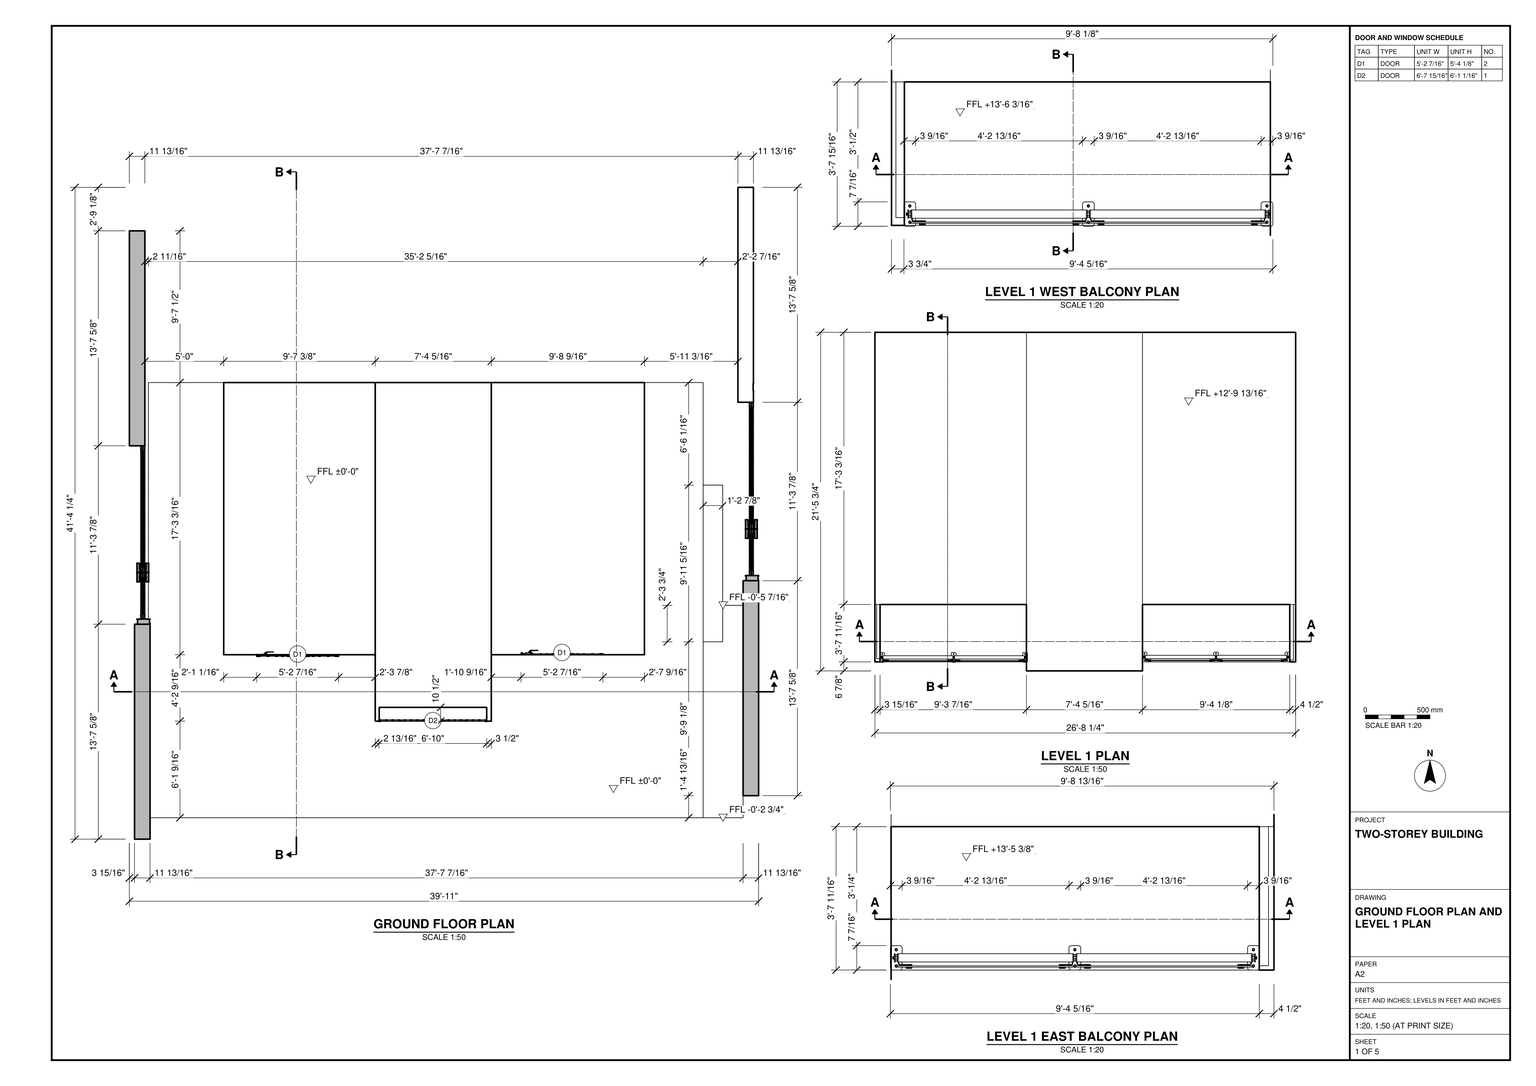
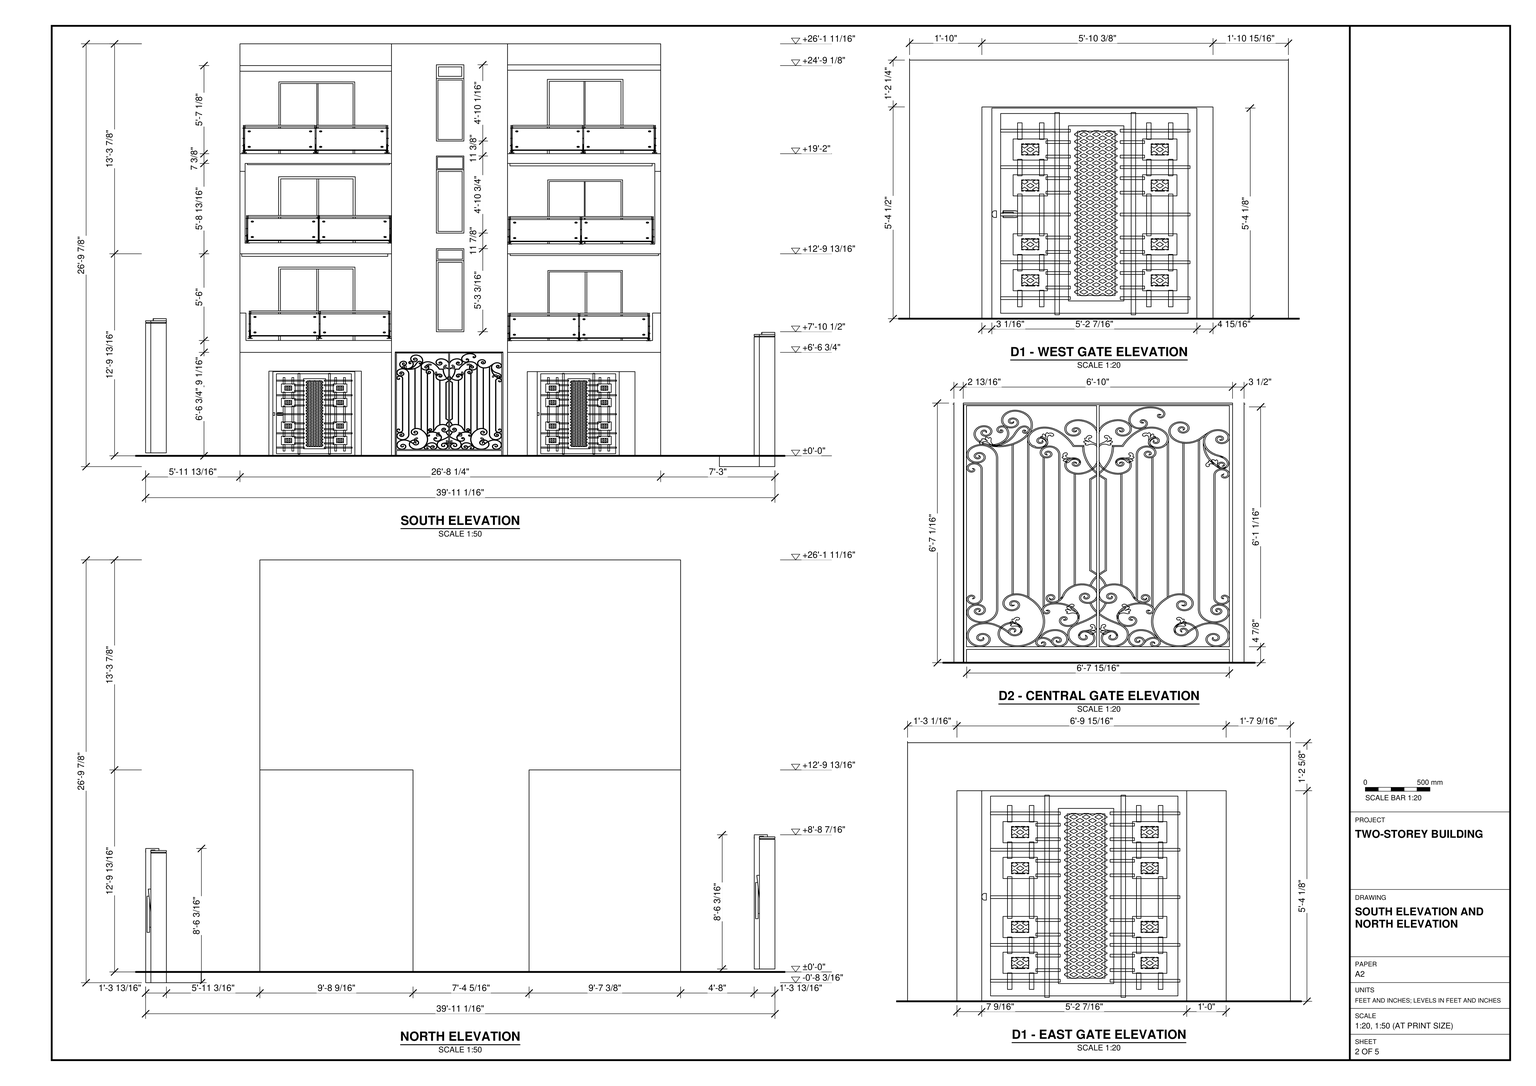
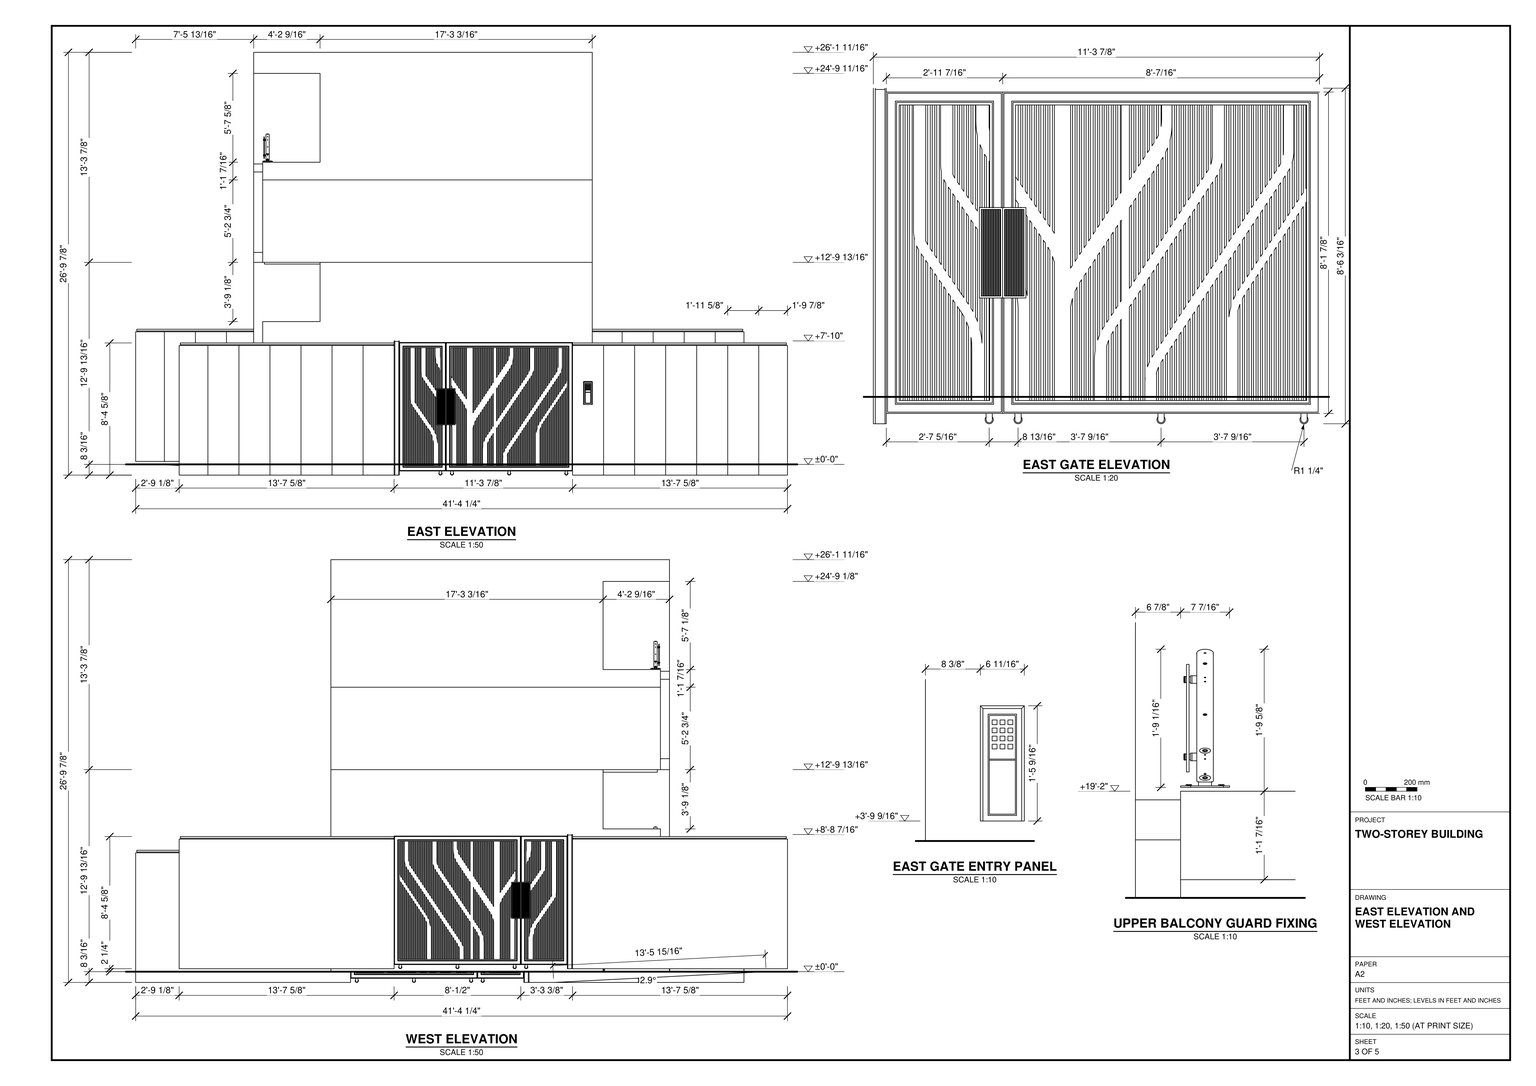
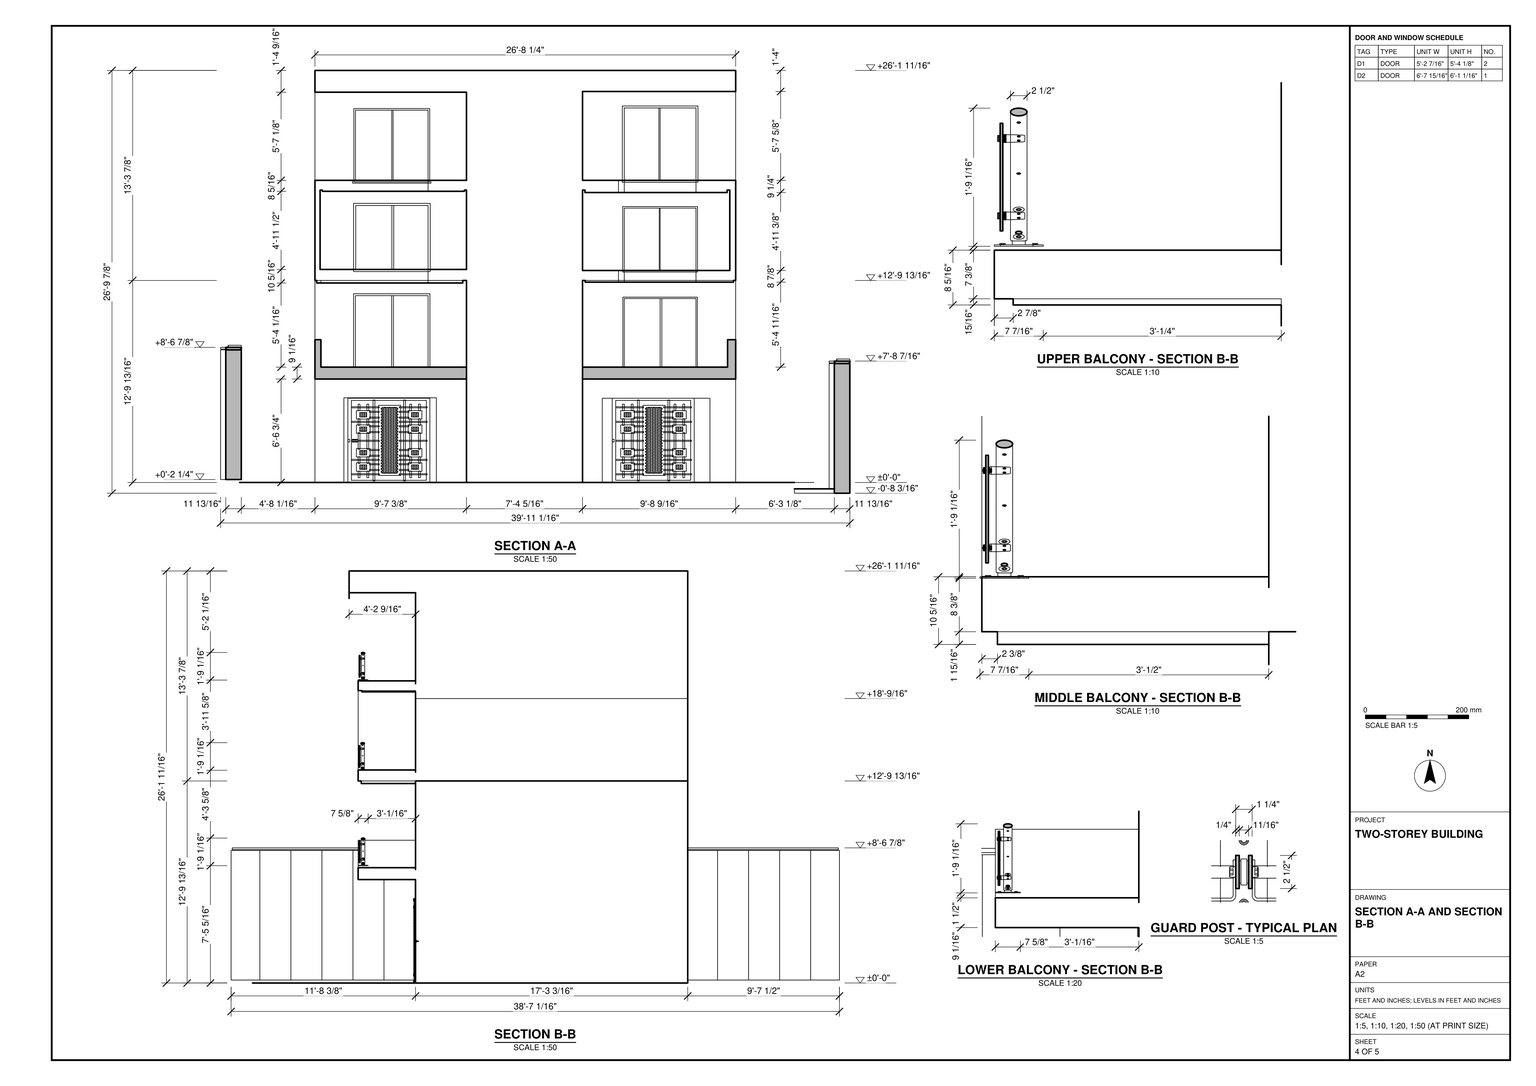
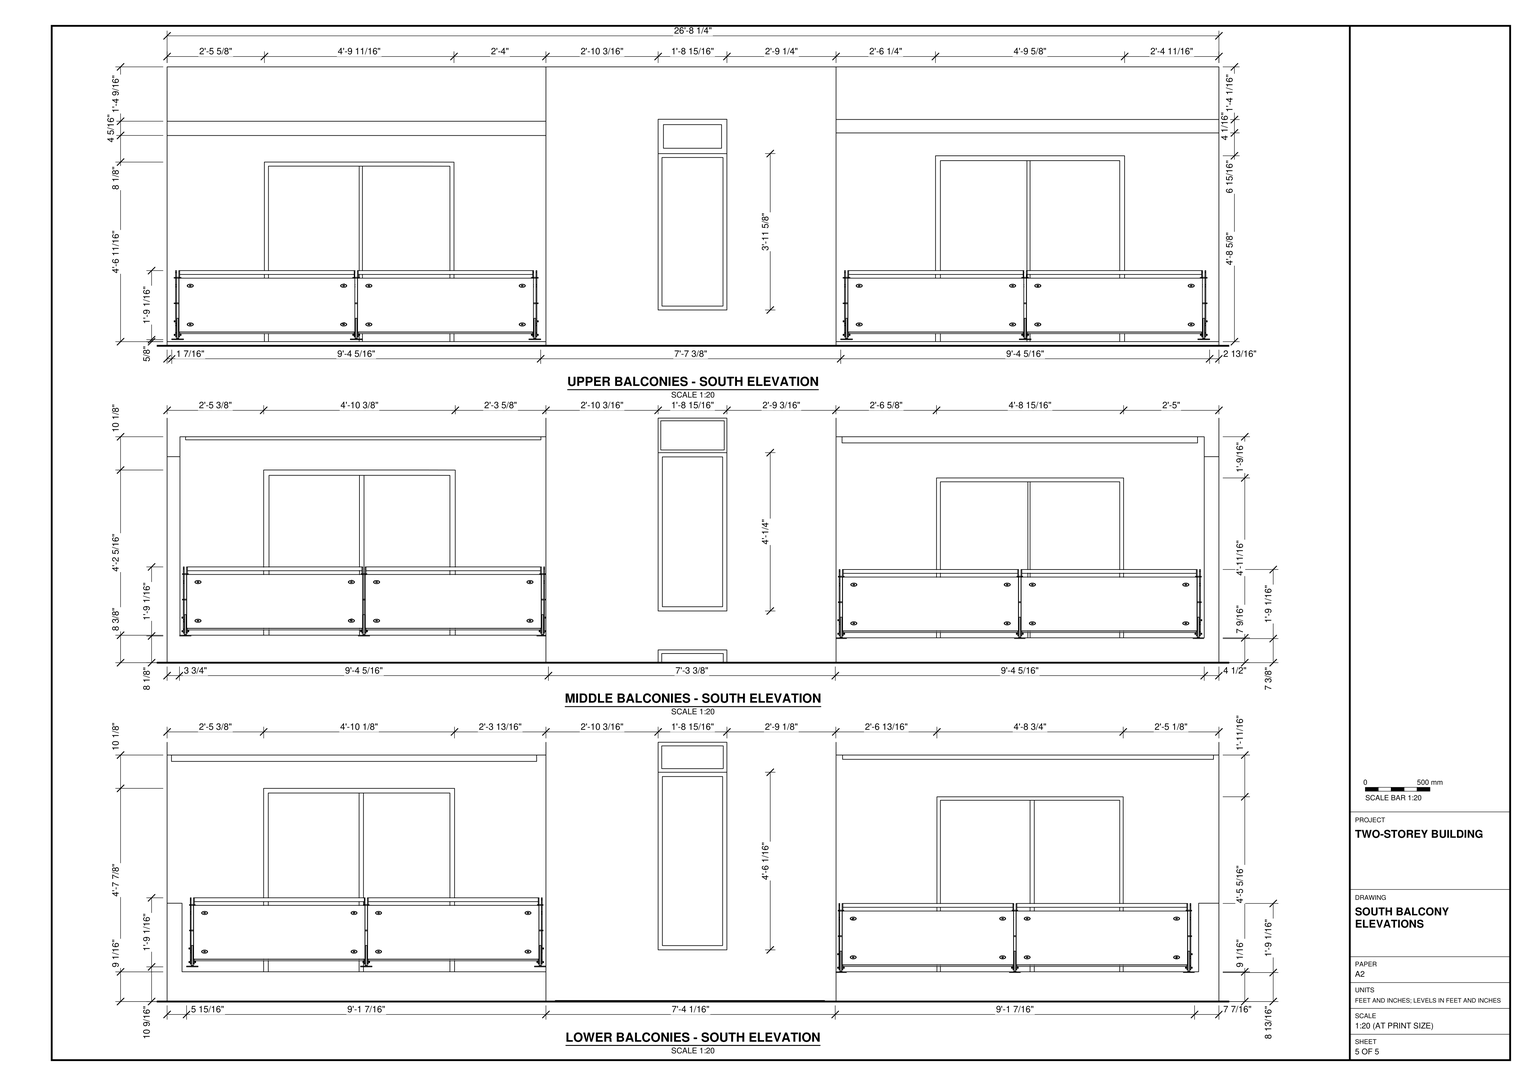
Build the two-storey building and its gated site in SketchUp using task_files/diagram_01.pdf. Work in feet and inches. Set out the complete model, including the side boundary walls, to an overall width of 39'-11 1/16", depth of 41'-4 1/4" and height of 26'-9 7/8". Use ±0'-0" for the ground floor and +12'-9 13/16" for Level 1.

Follow the plans for the building footprint, the projection of the central entrance bay and the clearances between the building and the boundary walls. Model the walls, floor and balcony slabs, openings and flat roof with their thicknesses as drawn. On the south face, place the wider central gate between the two matching entrance gates. Follow the south elevation for the three balcony tiers on either side of the central bay, including the glazed openings behind the guards and the narrow windows in the central bay. Use the balcony details for the glass panels, posts and fixings.

Model the east and west boundary walls with their gate openings in the positions shown in plan. Follow the side elevations for the unequal gate leaves, branching bar pattern and east entry panel. Keep shell elements, gates and any furniture or joinery pieces in separate groups or components, and use components for repeated parts. Decor and loose items, if shown, may be any suitable library components. Save one SketchUp model as output_files/two_storey_building_with_balconies_and_gated_side_walls.skp.

# SketchUp Ruby script. Lengths in inches.
U = 1.inch
M = Sketchup.active_model
def pt(a) = Geom::Point3d.new(a.map { |v| v * U })
def face(e, loops, mat)
  f = e.add_face(loops[0].map { |a| pt(a) })
  loops[1..].each { |l| e.add_face(l.map { |a| pt(a) }).erase! }
  f.material = f.back_material = mat if mat
  f
end
# faces: each face lists its corners as indices into pts; further lists are holes
def faces(e, pts, list, mat = nil) = list.each { |f| face(e, (f[0].is_a?(Array) ? f : [f]).map { |l| l.map { |i| pts[i] } }, mat) }
# xy, xz, yz: faces in a plane at the given z, y or x. An outline is a flat list of corners, or four numbers for a rectangle; further outlines are holes
def ring(l) = l.size == 4 ? [[l[0], l[1]], [l[2], l[1]], [l[2], l[3]], [l[0], l[3]]] : l.each_slice(2).to_a
def flat(e, list, mat, &to3) = list.each { |f| face(e, (f[0].is_a?(Array) ? f : [f]).map { |l| ring(l).map { |u, v| to3.(u, v) } }, mat) }
def xy(e, z, list, mat = nil) = flat(e, list, mat) { |x, y| [x, y, z] }
def xz(e, y, list, mat = nil) = flat(e, list, mat) { |x, z| [x, y, z] }
def yz(e, x, list, mat = nil) = flat(e, list, mat) { |y, z| [x, y, z] }
def lines(e, pts, list) = list.each { |a, b| e.add_line(pt(pts[a]), pt(pts[b])) }
# prism: a flat outline (further loops are holes) pulled along v
def prism(e, loops, v, mat = nil)
  f = face(e, loops, mat); d = Geom::Vector3d.new(v.map { |x| x * U })
  f.pushpull(f.normal.samedirection?(d) ? d.length : -d.length)
end
def box(e, o, s, mat = nil) = prism(e, [[o, [o[0] + s[0], o[1], o[2]], [o[0] + s[0], o[1] + s[1], o[2]], [o[0], o[1] + s[1], o[2]]]], [0, 0, s[2]], mat)
def at(x, y, z, deg = 0) = Geom::Transformation.translation(pt([x, y, z])) * Geom::Transformation.rotation(ORIGIN, Z_AXIS, deg.degrees)
def axes(o, x, y, z) = Geom::Transformation.new([*x, 0, *y, 0, *z, 0, *pt(o).to_a, 1])
def part(name) = M.definitions.add(name)
# library, detail: a bought-in or finely detailed component or shape, given as its bounding box
def library(name, o, s) = part(name).tap { |d| box(d.entities, o, s) }
def detail(e, o, s) = box(e.add_group.entities, o, s)
def put(e, d, t, mat = nil) = e.add_instance(d, t).tap { |i| i.material = mat if mat }
def group(e, t, mat = nil) = e.add_group.tap { |g| g.transformation = t; g.material = mat if mat }.entities
root = M.entities
M.materials.add("0-370-55720370副本4").color = [155, 133, 94]
M.materials.add("1").color = [35, 24, 16]
M.materials.add("Niraj_Hair_Dark").color = [109, 109, 109]
M.materials.add("[0009_Linen]").color = [250, 240, 230]
M.materials.add("[0028_AntiqueWhite]").color = [250, 235, 215]
M.materials.add("[Asphalt New]").color = [67, 60, 62]
M.materials.add("[Metal Corrugated Shiny]16").color = [144, 125, 78]
M.materials.add("[Translucent Glass Gray]").color = [128, 128, 128]
M.materials["[Translucent Glass Gray]"].alpha = 0.5
M.materials.add("主石材1").color = [201, 201, 201]
c1 = library("2.Gate",[0,0,0],[31.23,2.83,52.14])
c2 = library("Driveway gate",[0.2,-91.45,-1.97],[10.04,135.85,102.19])
c3 = part("组\#15")
xy(c3.entities,-0.2,[[111.54,0,274.3125,11.88]],"0-370-55720370副本4")
xy(c3.entities,0.98,[[[111.54,0,274.3125,11.88],[112.13,0.59,273.72,11.29]]],"0-370-55720370副本4")
xy(c3.entities,1.57,[[112.13,0.59,273.72,11.29]],"0-370-55720370副本4")
xz(c3.entities,0,[[111.54,-0.2,274.3125,0.98]],"0-370-55720370副本4")
xz(c3.entities,0.59,[[112.13,0.98,273.72,1.57]],"0-370-55720370副本4")
xz(c3.entities,11.29,[[112.13,0.98,273.72,1.57]],"0-370-55720370副本4")
xz(c3.entities,11.88,[[111.54,-0.2,274.3125,0.98]],"0-370-55720370副本4")
yz(c3.entities,111.54,[[0,-0.2,11.88,0.98]],"0-370-55720370副本4")
yz(c3.entities,112.13,[[0.59,0.98,11.29,1.57]],"0-370-55720370副本4")
yz(c3.entities,273.72,[[0.59,0.98,11.29,1.57]],"0-370-55720370副本4")
yz(c3.entities,274.3125,[[0,-0.2,11.88,0.98]],"0-370-55720370副本4")
c4 = part("组\#14")
xy(c4.entities,15.75,[[0.39,-1.18,6.3,0.79]],"[Metal Corrugated Shiny]16")
xy(c4.entities,16.14,[[0,-1.18,6.69,0.79]],"[Metal Corrugated Shiny]16")
xz(c4.entities,-1.18,[[0,0,0.39,0,0.39,15.75,6.3,15.75,6.3,0,6.69,0,6.69,16.14,0,16.14]],"[Metal Corrugated Shiny]16")
xz(c4.entities,0.79,[[0.39,15.75,0,16.14,6.69,16.14,6.3,15.75]],"[Metal Corrugated Shiny]16")
yz(c4.entities,0,[[-1.18,0,-1.18,16.14,0.79,16.14,-0.2,8.07]],"[Metal Corrugated Shiny]16")
yz(c4.entities,0.39,[[-1.18,0,-0.2,7.875,0.79,15.75,-1.18,15.75]],"[Metal Corrugated Shiny]16")
yz(c4.entities,6.3,[[-1.18,0,-1.18,15.75,0.79,15.75,-0.2,7.875]],"[Metal Corrugated Shiny]16")
yz(c4.entities,6.69,[[-1.18,0,-0.2,8.07,0.79,16.14,-1.18,16.14]],"[Metal Corrugated Shiny]16")
p = [[0.39,-0.2,7.875],[0,-0.2,8.07],[0,-1.18,0],[0.39,-1.18,0],[6.69,-0.2,8.07],[6.3,-0.2,7.875],
  [6.69,-1.18,0],[6.3,-1.18,0],[0.39,0.79,15.75],[6.3,0.79,15.75],[0,0.79,16.14],[6.69,0.79,16.14]]
faces(c4.entities,p,[[0,1,2],[0,2,3],[4,5,6],[6,5,7],[8,1,0],[4,9,5],[8,10,1],[11,9,4]],"[Metal Corrugated Shiny]16")
c5 = part("组\#1730")
xy(c5.entities,19.61,[[-11.8125,0,151.8125,11.8125]],"主石材1")
xy(c5.entities,84.78,[[137.15,9.84,143.05,11.8125]],"[Metal Corrugated Shiny]16")
xy(c5.entities,110.36,[[-11.8125,0,151.8125,11.8125]],"主石材1")
xz(c5.entities,0,[[-11.8125,19.61,151.8125,110.36]],"主石材1")
xz(c5.entities,11.8125,[[[-11.8125,19.61,151.8125,110.36],[136.75,69.03,143.45,85.18]],[136.75,69.03,136.75,85.18,143.45,85.18,143.45,69.03,143.05,69.03,143.05,84.78,137.15,84.78,137.15,69.03]],"主石材1")
yz(c5.entities,-11.8125,[[0,19.61,11.8125,110.36]],"主石材1")
yz(c5.entities,137.15,[[11.8125,69.03,11.8125,84.78,9.84,84.78]],"[Metal Corrugated Shiny]16")
yz(c5.entities,143.05,[[11.8125,69.03,9.84,84.78,11.8125,84.78]],"[Metal Corrugated Shiny]16")
yz(c5.entities,151.8125,[[0,19.61,11.8125,110.36]],"主石材1")
p = [[137.15,9.84,84.78],[143.05,9.84,84.78],[143.05,11.8125,69.03],[137.15,11.8125,69.03],[142.26,9.94,84],[137.93,9.94,84],
  [137.93,11.71,69.82],[142.26,11.71,69.82],[142.08,10.73,77.71],[138.12,10.73,77.71],[138.12,10.75,77.55],[138.12,11.69,70],
  [142.08,11.69,70],[142.08,10.75,77.55],[142.08,9.96,83.82],[138.12,9.96,83.82],[139.71,10.04,83.1875],[139.71,10.125,82.53],
  [140.45,10.125,82.53],[140.45,10.04,83.1875],[138.51,10.18,82.05],[138.51,10.27,81.4],[139.25,10.27,81.4],[139.25,10.18,82.05],
  [139.71,10.33,80.92],[139.71,10.41,80.26],[140.45,10.41,80.26],[140.45,10.33,80.92],[138.51,10.47,79.79],[138.51,10.55,79.13],
  [139.25,10.55,79.13],[139.25,10.47,79.79],[138.51,10.04,83.1875],[138.51,10.125,82.53],[139.25,10.125,82.53],[139.25,10.04,83.1875],
  [140.91,10.18,82.05],[140.91,10.27,81.4],[141.65,10.27,81.4],[141.65,10.18,82.05],[138.51,10.33,80.92],[138.51,10.41,80.26],
  [139.25,10.41,80.26],[139.25,10.33,80.92],[140.91,10.33,80.92],[140.91,10.41,80.26],[141.65,10.41,80.26],[141.65,10.33,80.92],
  [140.91,10.47,79.79],[140.91,10.55,79.13],[141.65,10.55,79.13],[141.65,10.47,79.79],[140.91,10.04,83.1875],[140.91,10.125,82.53],
  [141.65,10.125,82.53],[141.65,10.04,83.1875],[139.71,10.18,82.05],[139.71,10.27,81.4],[140.45,10.27,81.4],[140.45,10.18,82.05],
  [139.71,10.47,79.79],[139.71,10.55,79.13],[140.45,10.55,79.13],[140.45,10.47,79.79]]
faces(c5.entities,p,[[[0,1,2,3],[4,5,6,7]],[[5,4,7,6],[8,9,10,11,12,13]],[10,13,12,11],[13,10,9,8],[[14,8,9,15],[16,17,18,19],[20,21,22,23],[24,25,26,27],[28,29,30,31],[32,33,34,35],[36,37,38,39],[40,41,42,43],[44,45,46,47],[48,49,50,51],[52,53,54,55],[56,57,58,59],[60,61,62,63]],[29,28,31,30],[61,60,63,62],[49,48,51,50],
  [41,40,43,42],[25,24,27,26],[45,44,47,46],[21,20,23,22],[57,56,59,58],[37,36,39,38],[33,32,35,34],[17,16,19,18],
  [53,52,55,54]],"[Metal Corrugated Shiny]16")
put(c5.entities,c4,at(136.75,12.99,69.03))
c6 = part("组\#263")
p = [[151.8125,11.8125,19.61],[151.8125,11.8125,110.36],[128.1875,11.8125,19.61],[128.1875,11.8125,110.36],[104.57,11.8125,19.61],[104.57,11.8125,110.36],
  [80.94,11.8125,19.61],[80.94,11.8125,110.36],[57.32,11.8125,19.61],[57.32,11.8125,110.36],[33.7,11.8125,19.61],[33.7,11.8125,110.36],
  [10.08,11.8125,19.61],[10.08,11.8125,110.36]]
lines(c6.entities,p,[[0,1],[0,2],[2,3],[4,5],[6,7],[8,9],[10,11],[12,13],[10,12],[8,10],[6,8],[4,6],
  [2,4]])
put(c6.entities,c3,axes([263.35,0,111.9375],[-1,0,0],[0,1,0],[0,0,-1]))
put(c6.entities,c5,at(0,0,0))
c7 = part("组\#1715")
xy(c7.entities,-0.2,[[111.54,0,274.3125,11.88]],"0-370-55720370副本4")
xy(c7.entities,0.98,[[[111.54,0,274.3125,11.88],[112.13,0.59,273.72,11.29]]],"0-370-55720370副本4")
xy(c7.entities,1.57,[[112.13,0.59,273.72,11.29]],"0-370-55720370副本4")
xz(c7.entities,0,[[111.54,-0.2,274.3125,0.98]],"0-370-55720370副本4")
xz(c7.entities,0.59,[[112.13,0.98,273.72,1.57]],"0-370-55720370副本4")
xz(c7.entities,11.29,[[112.13,0.98,273.72,1.57]],"0-370-55720370副本4")
xz(c7.entities,11.88,[[111.54,-0.2,274.3125,0.98]],"0-370-55720370副本4")
yz(c7.entities,111.54,[[0,-0.2,11.88,0.98]],"0-370-55720370副本4")
yz(c7.entities,112.13,[[0.59,0.98,11.29,1.57]],"0-370-55720370副本4")
yz(c7.entities,273.72,[[0.59,0.98,11.29,1.57]],"0-370-55720370副本4")
yz(c7.entities,274.3125,[[0,-0.2,11.88,0.98]],"0-370-55720370副本4")
c8 = part("组\#17")
box(c8.entities,[-11.8125,0,19.61],[163.625,11.8125,90.75],"主石材1")
c9 = part("组\#18")
p = [[151.8125,11.8125,19.61],[151.8125,11.8125,110.36],[128.1875,11.8125,19.61],[128.1875,11.8125,110.36],[104.57,11.8125,19.61],[104.57,11.8125,110.36],
  [80.94,11.8125,19.61],[80.94,11.8125,110.36],[57.32,11.8125,19.61],[57.32,11.8125,110.36],[33.7,11.8125,19.61],[33.7,11.8125,110.36],
  [10.08,11.8125,19.61],[10.08,11.8125,110.36]]
lines(c9.entities,p,[[0,1],[0,2],[2,3],[4,5],[6,7],[8,9],[10,11],[12,13],[10,12],[8,10],[6,8],[4,6],
  [2,4]])
put(c9.entities,c7,axes([263.35,0,111.9375],[-1,0,0],[0,1,0],[0,0,-1]))
put(c9.entities,c8,at(0,0,0))
c10 = part("CỔNG+3+(4)")
put(c10.entities,c2,at(-0.2,91.48,1.78))
put(c10.entities,c6,axes([-5.71,287.7,-21.52],[0,-1,0],[1,0,0],[0,0,1.08753]))
put(c10.entities,c9,axes([-1.77,-151.77,-21.52],[0,1,0],[1,0,0],[0,0,1.08753]))
c11 = library("1",[60.35,22.11,0],[62.99,1.35,81.52])
c12 = library("Glass Railing\#8",[-1.57,-2.95,0],[99.14,5.9,36])
xy(root,0,[[14.48,16.29,436.8,16.29,436.8,347.6,392.11,347.6,392.11,140.4,275.52,140.4,275.52,89.84,272.03,89.84,272.03,100.34,190.19,100.34,190.19,89.84,187.18,89.84,187.18,140.4,71.83,140.4,71.83,347.6,14.48,347.6],[187.18,89.84,190.19,89.84,190.19,100.34,272.03,100.34,272.03,89.84,275.52,89.84,275.52,347.6,187.18,347.6],[71.83,140.4,187.18,347.6],[275.52,140.4,392.11,347.6],[436.8,150.23,451.6875,269.53]])
xy(root,78.6,[[190.19,89.84,272.03,100.34]])
xy(root,78.75,[[71.83,96.71,187.18,140.4],[275.52,96.71,392.11,140.4]])
xy(root,87.8125,[[76.38,96.71,187.18,140.4]])
xy(root,87.8125,[[275.52,96.71,385.94,140.4]],"[0009_Linen]")
xy(root,108.6875,[[71.83,96.71,76.38,140.4]])
xy(root,108.6875,[[385.94,96.71,392.11,140.4]],"[0009_Linen]")
xy(root,151.875,[[73.16,99.09,184.35,140.4]],"[0009_Linen]")
xy(root,152.5,[[277.52,98.03,390.44,140.4]])
xy(root,153.8125,[[71.83,96.71,71.83,140.4,73.16,140.4,73.16,99.09,184.35,99.09,184.35,140.4,187.18,140.4,187.18,96.71],[275.52,96.71,275.52,140.4,277.52,140.4,277.52,98.03,390.44,98.03,390.44,140.4,392.11,140.4,392.11,96.71],[71.83,140.4,187.18,347.6],[275.52,140.4,392.11,347.6]])
xy(root,161.39,[[275.52,96.71,387.64,140.4]],"[0009_Linen]")
xy(root,162.18,[[75.74,96.71,187.18,140.4]])
xy(root,220.74,[[277.35,98.28,385.6,140.4]])
xy(root,221.68,[[77.46,99.59,185.65,140.4]],"[0009_Linen]")
xy(root,222.61,[[275.52,96.71,275.52,140.4,277.35,140.4,277.35,98.28,385.6,98.28,385.6,140.4,387.64,140.4,387.64,96.71]])
xy(root,222.61,[[75.74,96.71,75.74,140.4,77.46,140.4,77.46,99.59,185.65,99.59,185.65,140.4,187.18,140.4,187.18,96.71]],"[0009_Linen]")
xy(root,230.02,[[71.83,96.71,187.18,140.4]])
xy(root,230.02,[[275.52,96.71,392.11,140.4]],"[0009_Linen]")
xy(root,297.12,[[71.83,89.84,187.18,140.4]],"[0009_Linen]")
xy(root,297.66,[[275.52,89.84,392.11,140.4]])
xy(root,313.6875,[[71.83,89.84,187.18,347.6],[187.18,89.84,275.52,347.6],[275.52,89.84,392.11,347.6]])
xz(root,89.84,[[[187.18,0,190.19,0,190.19,78.6,272.03,78.6,272.03,0,275.52,0,275.52,313.6875,187.18,313.6875],[221.34,94.49,242.29,157.71],[221.34,169.56,242.29,228.29],[221.34,239.65,242.29,297.73]]])
xz(root,89.84,[[71.83,297.12,187.18,313.6875],[275.52,297.66,392.11,313.6875]],"Niraj_Hair_Dark")
xz(root,89.84,[[71.83,292.78,187.18,297.12],[275.52,293.57,392.11,297.66]],"[0009_Linen]")
xz(root,89.84,[[[221.34,94.49,242.29,148.57],[222.64,95.79,240.99,147.27]],[[221.34,148.57,242.29,157.71],[222.45,149.67,241.18,156.6]],[[221.34,169.56,242.29,217.78],[222.64,170.85,240.99,216.48]],[[221.34,217.78,242.29,228.29],[222.15,218.59,241.47,227.48]],[[221.34,239.65,242.29,287.27],[222.52,240.83,241.11,286.09]],
  [[221.34,287.27,242.29,297.73],[222.97,288.89,240.66,296.1]]],"[Asphalt New]")
xz(root,89.84,[[222.64,95.79,240.99,147.27],[222.45,149.67,241.18,156.6],[222.64,170.85,240.99,216.48],[222.15,218.59,241.47,227.48],[222.52,240.83,241.11,286.09],
  [222.97,288.89,240.66,296.1]],"[Translucent Glass Gray]")
xz(root,96.71,[[71.83,78.75,187.18,78.75,187.18,87.8125,76.38,87.8125,76.38,108.6875,71.83,108.6875],[275.52,78.75,392.11,78.75,392.11,108.6875,385.94,108.6875,385.94,87.8125,275.52,87.8125],[71.83,153.8125,187.18,153.8125,187.18,162.18,75.74,162.18,75.74,216.55,71.83,216.55],[275.52,153.8125,392.11,153.8125,392.11,216.55,387.64,216.55,387.64,161.39,275.52,161.39],[71.83,216.55,75.74,216.55,75.74,222.61,187.18,222.61,187.18,230.02,71.83,230.02],
  [387.64,216.55,392.11,216.55,392.11,230.02,275.52,230.02,275.52,222.61,387.64,222.61]],"[0009_Linen]")
xz(root,98.03,[[277.52,152.5,390.44,153.8125]])
xz(root,98.28,[[277.35,220.74,385.6,222.61]])
xz(root,99.09,[[73.16,151.875,184.35,153.8125]],"[0009_Linen]")
xz(root,99.59,[[77.46,221.68,185.65,222.61]],"[0009_Linen]")
xz(root,100.34,[[190.19,0,272.03,78.6]],"[0028_AntiqueWhite]")
xz(root,140.4,[[101.22,86.4,159.36,87.8125],[306.25,86.76,362.96,87.8125],[73.16,151.875,76.38,153.8125],[76.38,151.875,157.95,153.8125],[157.95,151.875,184.35,153.8125],
  [277.52,152.5,302.88,153.8125],[302.88,152.5,307.3,153.8125],[307.3,152.5,361.91,153.8125],[361.91,152.5,390.44,153.8125],[302.88,153.8125,307.3,153.8125,307.3,160.21,306.12,160.21,306.12,161.39,302.88,161.39],
  [307.3,153.8125,361.91,160.21],[306.12,160.21,307.3,161.39],[307.3,160.21,361.91,161.39],[361.91,160.21,363.08,161.39],[101.23,160.55,157.95,162.18],
  [157.95,160.55,159.57,162.18],[302.88,220.74,307.3,220.74,307.3,228.54,305.82,228.54,305.82,230.02,302.88,230.02],[307.3,220.74,361.91,228.54],[100.5,227.83,157.95,227.83,157.95,228.78,101.45,228.78,101.45,230.02,100.5,230.02],[157.95,227.83,160.13,227.83,160.13,230.02,159.1875,230.02,159.1875,228.78,157.95,228.78],
  [305.82,228.54,307.3,230.02],[307.3,228.54,361.91,230.02],[361.91,228.54,363.38,230.02],[101.45,228.78,157.95,230.02],[157.95,228.78,159.1875,230.02]])
xz(root,140.4,[[71.83,0,93.85,0,93.85,64.47,164.22,64.47,164.22,0,187.18,0,187.18,78.75,71.83,78.75],[275.52,0,290.54,0,290.54,64.13,372.54,64.13,372.54,0,392.11,0,392.11,78.75,275.52,78.75],[76.38,87.8125,101.22,87.8125,101.22,143.66,159.36,143.66,159.36,87.8125,187.18,87.8125,187.18,153.8125,184.35,153.8125,184.35,151.875,73.16,151.875,73.16,153.8125,71.83,153.8125,71.83,108.6875,76.38,108.6875],[275.52,87.8125,306.25,87.8125,306.25,141.09,362.96,141.09,362.96,87.8125,385.94,87.8125,385.94,108.6875,392.11,108.6875,392.11,153.8125,390.44,153.8125,390.44,152.5,277.52,152.5,277.52,153.8125,275.52,153.8125],[275.52,161.39,306.12,161.39,306.12,210.07,363.08,210.07,363.08,161.39,387.64,161.39,387.64,222.61,385.6,222.61,385.6,220.74,277.35,220.74,277.35,222.61,275.52,222.61],
  [75.74,162.18,101.23,162.18,101.23,212.49,151.55,212.49,159.57,212.47,159.57,162.18,187.18,162.18,187.18,222.61,185.65,222.61,185.65,221.68,77.46,221.68,77.46,222.61,75.74,222.61],[71.83,230.02,101.45,230.02,101.45,284.7,150.0625,284.7,159.1875,284.68,159.1875,230.02,187.18,230.02,187.18,297.12,71.83,297.12],[275.52,230.02,305.82,230.02,305.82,286.6,363.38,286.6,363.38,230.02,392.11,230.02,392.11,297.66,275.52,297.66]],"[0009_Linen]")
xz(root,140.4,[[101.22,87.8125,102.63,87.8125,102.63,142.25,157.95,142.25,157.95,87.8125,159.36,87.8125,159.36,143.66,101.22,143.66],[130.29,87.8125,131.62,142.25],[306.25,87.8125,307.3,87.8125,307.3,140.04,361.91,140.04,361.91,87.8125,362.96,87.8125,362.96,141.09,306.25,141.09],[334.6,87.8125,335.88,140.04],[306.12,161.39,307.3,161.39,307.3,208.89,361.91,208.89,361.91,161.39,363.08,161.39,363.08,210.07,306.12,210.07],
  [333.9375,161.39,334.6,208.89],[101.23,162.18,102.86,162.18,102.86,210.86,151.54,210.86,157.95,210.85,157.95,162.18,159.57,162.18,159.57,212.47,151.55,212.49,101.23,212.49],[130.4,162.18,131.79,210.86],[101.45,230.02,102.6875,230.02,102.6875,283.46,150.0625,283.46,157.95,283.4375,157.95,230.02,159.1875,230.02,159.1875,284.68,150.0625,284.7,101.45,284.7],[130.32,230.02,131.31,283.46],
  [305.82,230.02,307.3,230.02,307.3,285.125,361.91,285.125,361.91,230.02,363.38,230.02,363.38,286.6,305.82,286.6],[333.65,230.02,334.6,285.125]],"[Asphalt New]")
xz(root,140.4,[[93.85,0,164.22,64.47],[290.54,0,372.54,64.13],[102.63,87.8125,130.29,142.25],[131.62,87.8125,157.95,142.25],[307.3,87.8125,334.6,140.04],
  [335.88,87.8125,361.91,140.04],[307.3,161.39,333.9375,208.89],[334.6,161.39,361.91,208.89],[102.86,162.18,130.4,210.86],[131.79,162.18,157.95,162.18,157.95,210.85,151.54,210.86,131.79,210.86],
  [102.6875,230.02,130.32,283.46],[131.31,230.02,157.95,230.02,157.95,283.4375,150.0625,283.46,131.31,283.46],[307.3,230.02,333.65,285.125],[334.6,230.02,361.91,285.125]],"[Translucent Glass Gray]")
xz(root,347.6,[[187.18,0,187.18,153.8125,71.83,153.8125,71.83,313.6875,392.11,313.6875,392.11,153.8125,275.52,153.8125,275.52,0],[71.83,0,187.18,153.8125],[275.52,0,392.11,153.8125]])
yz(root,71.83,[[140.4,0,140.4,78.75,96.71,78.75,96.71,108.6875,140.4,108.6875,140.4,153.8125,347.6,153.8125,347.6,0],[96.71,153.8125,347.6,216.55],[96.71,216.55,96.71,230.02,140.4,230.02,140.4,297.12,89.84,297.12,89.84,313.6875,347.6,313.6875,347.6,216.55]],"[0009_Linen]")
yz(root,73.16,[[99.09,151.875,140.4,153.8125]])
yz(root,75.74,[[96.71,162.18,140.4,222.61]])
yz(root,76.38,[[96.71,87.8125,140.4,108.6875]])
yz(root,77.46,[[99.59,221.68,140.4,222.61]])
yz(root,184.35,[[99.09,151.875,140.4,153.8125]])
yz(root,185.65,[[99.59,221.68,140.4,222.61]])
yz(root,187.18,[[89.84,0,140.4,78.75],[140.4,0,140.4,78.75,96.71,78.75,96.71,87.8125,140.4,87.8125,140.4,153.8125,347.6,153.8125,347.6,0],[89.84,78.75,96.71,87.8125],[89.84,87.8125,140.4,153.8125],[89.84,153.8125,96.71,162.18],
  [89.84,162.18,140.4,222.61],[89.84,222.61,96.71,228.71],[89.84,228.71,89.84,297.12,140.4,297.12,140.4,230.02,96.71,230.02,96.71,228.71]])
yz(root,190.19,[[89.84,0,100.34,78.6]])
yz(root,272.03,[[89.84,0,100.34,78.6]])
yz(root,275.52,[[89.84,0,140.4,78.75],[140.4,0,347.6,0,347.6,153.8125,140.4,153.8125,140.4,87.8125,96.71,87.8125,96.71,78.75,140.4,78.75],[89.84,78.75,96.71,87.8125],[89.84,87.8125,140.4,153.8125],[89.84,153.8125,96.71,161.39],
  [89.84,161.39,140.4,222.61],[89.84,222.61,96.71,228.71],[89.84,228.71,96.71,228.71,96.71,230.02,140.4,230.02,140.4,297.66,89.84,297.66]])
yz(root,277.35,[[98.28,220.74,140.4,222.61]])
yz(root,277.52,[[98.03,152.5,140.4,153.8125]])
yz(root,385.6,[[98.28,220.74,140.4,222.61]])
yz(root,385.94,[[96.71,87.8125,140.4,108.6875]])
yz(root,387.64,[[96.71,161.39,140.4,222.61]])
yz(root,390.44,[[98.03,152.5,140.4,153.8125]])
yz(root,392.11,[[140.4,0,347.6,0,347.6,153.8125,140.4,153.8125,140.4,108.6875,96.71,108.6875,96.71,78.75,140.4,78.75],[96.71,153.8125,347.6,216.55],[96.71,216.55,347.6,216.55,347.6,313.6875,89.84,313.6875,89.84,297.66,140.4,297.66,140.4,230.02,96.71,230.02]],"[0009_Linen]")
p = [[436.8,16.29,0],[467.2,16.29,0],[467.2,178.01,-8.1875],[436.8,178.01,-8.1875],[157.95,140.4,153.8125],[157.95,140.4,160.55],
  [157.95,140.4,221.68],[157.95,140.4,227.83]]
faces(root,p,[[0,1,2,3]])
lines(root,p,[[4,5],[6,7]])
put(root,c1,axes([96.88,139.18,0],[1.99875,0,0],[0,1.23,0],[0,0,1.23]))
put(root,c1,axes([298.11,140.4,0],[1.99875,0,0],[0,1.23,0],[0,0,1.23]))
put(root,c10,at(468.97,196.71,-8))
put(root,c10,at(5.71,163.58,2.4375))
put(root,c11,axes([111.44,68.17,0],[1.30202,0,0],[0,0.97,0],[0,0,0.97]))
put(root,c12,axes([79.5,100.52,89.3125],[1.10357,0,0],[0,1.2878,0],[0,0,0.5843]))
put(root,c12,axes([277.01,100.36,87.58],[1.10357,0,0],[0,1.2878,0],[0,0,0.5843]))
put(root,c12,axes([277.09,100.4375,161.16],[1.13294,0,0],[0,1.26119,0],[0,0,0.5843]))
put(root,c12,axes([77.39,100.15,161.95],[1.13294,0,0],[0,1.26119,0],[0,0,0.5843]))
put(root,c12,axes([75.03,100.4375,230.61],[1.13294,0,0],[0,1.26119,0],[0,0,0.5843]))
put(root,c12,axes([278.73,100.4375,230.61],[1.13294,0,0],[0,1.26119,0],[0,0,0.5843]))
